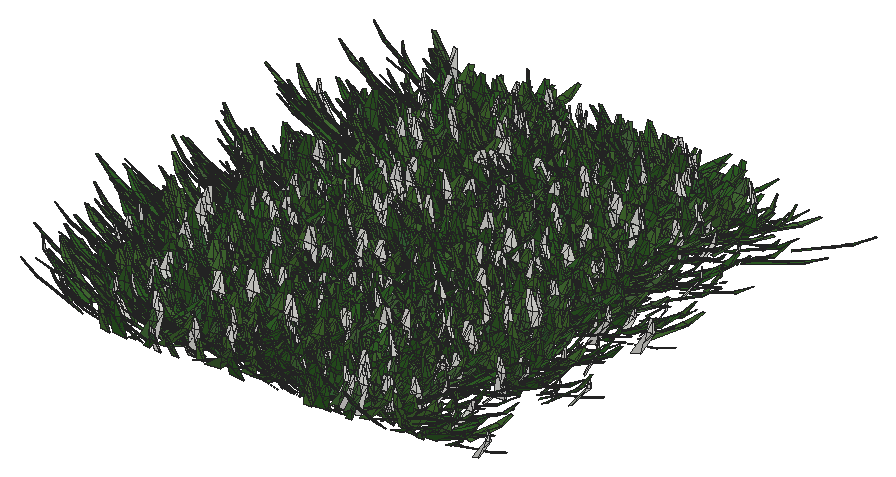
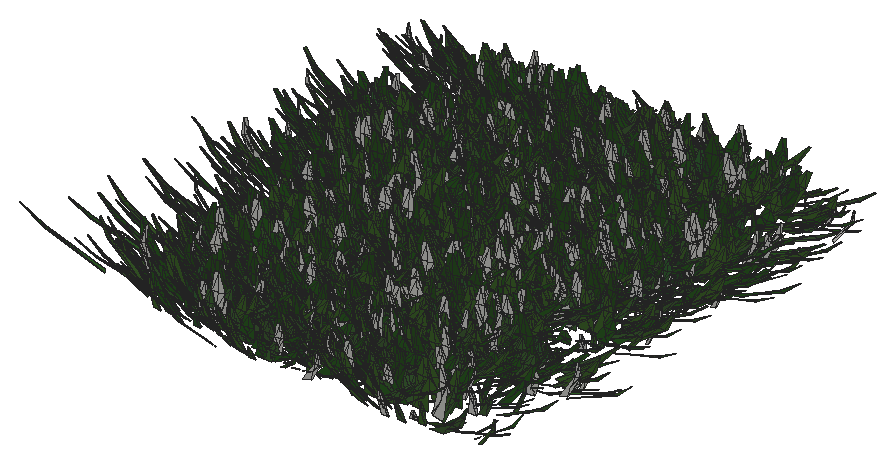
# SketchUp Ruby script. Lengths in inches.
U = 1.inch
M = Sketchup.active_model
def pt(a) = Geom::Point3d.new(a.map { |v| v * U })
def face(e, loops, mat)
  f = e.add_face(loops[0].map { |a| pt(a) })
  loops[1..].each { |l| e.add_face(l.map { |a| pt(a) }).erase! }
  f.material = f.back_material = mat if mat
  f
end
# faces: each face lists its corners as indices into pts; further lists are holes
def faces(e, pts, list, mat = nil) = list.each { |f| face(e, (f[0].is_a?(Array) ? f : [f]).map { |l| l.map { |i| pts[i] } }, mat) }
# xy, xz, yz: faces in a plane at the given z, y or x. An outline is a flat list of corners, or four numbers for a rectangle; further outlines are holes
def ring(l) = l.size == 4 ? [[l[0], l[1]], [l[2], l[1]], [l[2], l[3]], [l[0], l[3]]] : l.each_slice(2).to_a
def flat(e, list, mat, &to3) = list.each { |f| face(e, (f[0].is_a?(Array) ? f : [f]).map { |l| ring(l).map { |u, v| to3.(u, v) } }, mat) }
def xy(e, z, list, mat = nil) = flat(e, list, mat) { |x, y| [x, y, z] }
def xz(e, y, list, mat = nil) = flat(e, list, mat) { |x, z| [x, y, z] }
def yz(e, x, list, mat = nil) = flat(e, list, mat) { |y, z| [x, y, z] }
def lines(e, pts, list) = list.each { |a, b| e.add_line(pt(pts[a]), pt(pts[b])) }
# prism: a flat outline (further loops are holes) pulled along v
def prism(e, loops, v, mat = nil)
  f = face(e, loops, mat); d = Geom::Vector3d.new(v.map { |x| x * U })
  f.pushpull(f.normal.samedirection?(d) ? d.length : -d.length)
end
def box(e, o, s, mat = nil) = prism(e, [[o, [o[0] + s[0], o[1], o[2]], [o[0] + s[0], o[1] + s[1], o[2]], [o[0], o[1] + s[1], o[2]]]], [0, 0, s[2]], mat)
def at(x, y, z, deg = 0) = Geom::Transformation.translation(pt([x, y, z])) * Geom::Transformation.rotation(ORIGIN, Z_AXIS, deg.degrees)
def axes(o, x, y, z) = Geom::Transformation.new([*x, 0, *y, 0, *z, 0, *pt(o).to_a, 1])
def part(name) = M.definitions.add(name)
# library, detail: a bought-in or finely detailed component or shape, given as its bounding box
def library(name, o, s) = part(name).tap { |d| box(d.entities, o, s) }
def detail(e, o, s) = box(e.add_group.entities, o, s)
def put(e, d, t, mat = nil) = e.add_instance(d, t).tap { |i| i.material = mat if mat }
def group(e, t, mat = nil) = e.add_group.tap { |g| g.transformation = t; g.material = mat if mat }.entities
root = M.entities
M.materials.add("Material10").color = [48, 100, 38]
M.materials.add("Material3").color = [68, 110, 58]
M.materials.add("Material4").color = [48, 90, 38]
M.materials.add("Material5").color = [68, 110, 48]
M.materials.add("Material6").color = [48, 90, 48]
M.materials.add("Material7").color = [58, 110, 58]
M.materials.add("Material8").color = [58, 90, 38]
M.materials.add("Material9").color = [68, 100, 58]
c1 = part("grass00")
p = [[-0.6875,0.15,0],[-0.56,0.08,5.52],[-0.04,0.03,2.76],[0.48,-0.02,0],[0.35,-0.02,5.52],[-0.1,-0.14,5.52],
  [-0.12,0.65,8.37],[-0.42,0.65,8.37]]
faces(c1.entities,p,[[0,1,2,3],[3,2,4],[1,5,2],[5,4,2],[1,6,5],[4,5,6],[7,6,1]])
c2 = part("Group16\#1")
put(c2.entities,c1,axes([1.44,-0.61,-0.01],[0.05352,0.12609,0],[-0.10704,0.04543,0.07239],[0.06664,-0.02828,0.11628]),"Material6")
put(c2.entities,c1,axes([0.76,-0.15,-0.01],[0.04676,0.24062,0],[-0.23162,0.04501,0.06642],[0.0652,-0.01267,0.23595]),"Material3")
put(c2.entities,c1,axes([0.79,0.01,-0.01],[-0.00606,0.34651,0],[-0.34381,-0.00602,0.0432],[0.04319,0.00076,0.34386]))
put(c2.entities,c1,axes([1,0.23,-0.01],[-0.07192,0.31144,0],[-0.28722,-0.06632,0.1236],[0.12043,0.02781,0.29478]),"Material5")
put(c2.entities,c1,axes([1.66,0.77,-0.01],[-0.13828,0.29651,0],[-0.21551,-0.1005,0.22471],[0.20365,0.09498,0.23779]),"Material10")
put(c2.entities,c1,axes([0.6875,0.52,-0.01],[-0.18126,0.24051,0],[-0.22746,-0.17142,0.09788],[0.07817,0.05891,0.28481]),"Material5")
put(c2.entities,c1,axes([0.68,0.78,-0.01],[-0.215,0.18688,0],[-0.12385,-0.14248,0.21334],[0.13995,0.16101,0.18878]),"Material3")
put(c2.entities,c1,axes([0.56,1,-0.01],[-0.13756,0.07624,0],[-0.06159,-0.11112,0.0927],[0.04494,0.08108,0.12705]),"Material5")
put(c2.entities,c1,axes([0.2,0.64,-0.01],[-0.23729,0.07254,0],[-0.05711,-0.18681,0.153],[0.04473,0.14632,0.19535]),"Material10")
put(c2.entities,c1,axes([0.0625,0.72,-0.01],[-0.28874,0.02525,0],[-0.02179,-0.24916,0.14647],[0.01276,0.14591,0.25012]),"Material3")
put(c2.entities,c1,axes([-0.08,0.62,-0.01],[-0.34089,-0.04187,0],[0.03255,-0.26504,0.216],[-0.02633,0.21439,0.26703]),"Material10")
put(c2.entities,c1,axes([-0.34,0.98,-0.01],[-0.14314,-0.0493,0],[0.04397,-0.12769,0.06843],[-0.02228,0.0647,0.13505]),"Material10")
put(c2.entities,c1,axes([-0.87,1.45,-0.01],[-0.23488,-0.14114,0],[0.13761,-0.22901,0.06087],[-0.03135,0.05217,0.26717]))
put(c2.entities,c1,axes([-0.72,0.77,-0.01],[-0.14208,-0.13251,0],[0.07209,-0.0773,0.16301],[-0.11118,0.11922,0.1057]),"Material10")
put(c2.entities,c1,axes([-0.62,0.43,-0.01],[-0.14845,-0.21203,0],[0.18654,-0.13061,0.12304],[-0.10079,0.07057,0.22772]),"Material3")
put(c2.entities,c1,axes([-0.68,0.29,-0.01],[-0.13639,-0.32136,0],[0.31723,-0.13464,0.05579],[-0.05136,0.0218,0.34462]),"Material4")
put(c2.entities,c1,axes([-0.64,0.125,-0.01],[-0.0458,-0.23569,0],[0.22124,-0.043,0.08276],[-0.08124,0.01579,0.22538]),"Material7")
put(c2.entities,c1,axes([-1.6,-0.03,-0.01],[0.00576,-0.32897,0],[0.27526,0.00482,0.18018],[-0.18015,-0.00315,0.2753]),"Material5")
put(c2.entities,c1,axes([-1.36,-0.31,-0.01],[0.05718,-0.24765,0],[0.18172,0.04196,0.17267],[-0.16825,-0.03885,0.1865]),"Material10")
put(c2.entities,c1,axes([-1.54,-0.72,-0.01],[0.06537,-0.14017,0],[0.13555,0.06321,0.03939],[-0.0357,-0.01665,0.14956]))
put(c2.entities,c1,axes([-1.19,-0.9,-0.01],[0.09597,-0.12735,0],[0.11214,0.08451,0.07557],[-0.06035,-0.04548,0.14042]),"Material9")
put(c2.entities,c1,axes([-0.47,-0.54,-0.01],[0.11588,-0.10072,0],[0.0618,0.0711,0.12124],[-0.07953,-0.0915,0.0942]))
put(c2.entities,c1,axes([-0.47,-0.84,-0.01],[0.11927,-0.0661,0],[0.06603,0.11913,0.00646],[-0.00313,-0.00565,0.13621]),"Material5")
put(c2.entities,c1,axes([-0.38,-1.24,-0.01],[0.28037,-0.08571,0],[0.0618,0.20215,0.20315],[-0.05939,-0.19428,0.21139]),"Material9")
put(c2.entities,c1,axes([-0.06,-0.66,-0.01],[0.22719,-0.01987,0],[0.01247,0.14255,0.17758],[-0.01547,-0.17691,0.1431]),"Material8")
put(c2.entities,c1,axes([0.11,-0.89,-0.01],[0.14882,0.01828,0],[-0.01058,0.08611,0.12229],[0.01491,-0.12138,0.08676]),"Material6")
put(c2.entities,c1,axes([0.25,-0.72,-0.01],[0.20481,0.07053,0],[-0.06206,0.18022,0.10291],[0.03351,-0.0973,0.1906]),"Material6")
put(c2.entities,c1,axes([0.85,-1.42,-0.01],[0.16481,0.09904,0],[-0.09472,0.15762,0.05616],[0.02893,-0.04814,0.18389]),"Material5")
put(c2.entities,c1,axes([1.01,-1.09,-0.01],[0.21858,0.20385,0],[-0.17495,0.1876,0.15339],[0.10462,-0.11218,0.25652]),"Material10")
put(c2.entities,c1,axes([1.01,-0.71,-0.01],[0.08733,0.12473,0],[-0.06445,0.04512,0.13037],[0.1068,-0.07477,0.07867]),"Material6")
c3 = part("Group15\#1")
put(c3.entities,c2,at(0,0,0))
c4 = part("3darcstudiotree_grass00\#1")
put(c4.entities,c3,at(0,0,0))
put(root,c4,axes([859.57,954.71,0],[0.26147,-1.07741,0],[4.77538,0.07243,-0.04584],[0.20115,0.00305,1.3146]))
put(root,c4,axes([859.86,942.64,0],[-0.00527,-1.07979,0],[5.08619,-0.00155,-0.02113],[0.09419,-0.00003,1.41674]))
put(root,c4,axes([858.4,937.72,0],[3.80252,-0.21307,0],[0.8211,0.91584,-0.01015],[0.01463,0.01631,1.54623]))
put(root,c4,axes([858.36,939.11,0],[-1.38358,0.95904,0],[-3.87916,-0.34977,-0.00809],[-0.05318,-0.0048,1.80065]))
put(root,c4,axes([860.09,972.71,0],[-2.64683,-0.75591,0],[3.71627,-0.81329,-0.03006],[0.12697,-0.02779,1.73276]))
put(root,c4,axes([859.0625,943.74,0],[3.22127,-0.6295,0],[2.94777,0.94277,-0.00613],[0.02206,0.00705,1.74641]))
put(root,c4,axes([858.26,952.51,0],[0.12956,0.95583,0],[-3.83664,0.0325,-0.00216],[-0.01582,0.00013,1.758]))
put(root,c4,axes([859.75,968.45,0],[0.29566,-0.96452,0],[4.47879,0.08581,-0.05496],[0.37486,0.00718,1.9204]))
put(root,c4,axes([860.07,946.03,0],[-0.81018,-1.00031,0],[4.10104,-0.2076,-0.04711],[0.26622,-0.01348,1.50792]))
put(root,c4,axes([859.15,960.93,0],[3.64126,-0.56822,0],[2.32111,0.92964,-0.03499],[0.12777,0.05117,1.88939]))
put(root,c4,axes([859.51,949.74,0],[2.71786,-0.72349,0],[3.02088,0.70927,-0.02466],[0.11069,0.02599,1.59511]))
put(root,c4,axes([859.33,940.95,0],[-3.07818,0.70756,0],[-3.19663,-0.86917,-0.0061],[-0.02564,-0.00697,1.83281]))
put(root,c4,axes([859.26,936.04,0],[-1.05333,1.02923,0],[-4.06109,-0.25976,-0.04208],[-0.23965,-0.01533,1.54007]))
put(root,c4,axes([860.87,948.46,0],[-0.35317,-0.93176,0],[5.0183,-0.11888,-0.03587],[0.18182,-0.00431,1.60406]))
put(root,c4,axes([859.13,929.75,0],[0.93736,0.93245,0],[-4.81106,0.30227,-0.04255],[-0.20854,0.0131,1.5668]))
put(root,c4,axes([859.34,963.21,0],[4.77949,0.09804,0],[-0.30213,0.92053,-0.01884],[-0.00915,0.02789,1.37151]))
put(root,c4,axes([859.22,962.51,0],[3.18507,0.78996,0],[-2.86494,0.72195,-0.02475],[-0.11175,0.02816,1.62992]))
put(root,c4,axes([859.48,935.36,0],[4.28562,0.46278,0],[-1.51887,0.87911,-0.02193],[-0.0534,0.03091,1.47013]))
put(root,c4,axes([860.44,926.77,0],[3.286,-0.8357,0],[2.84385,0.69888,-0.02297],[0.11018,0.02708,1.67632]))
put(root,c4,axes([860.38,933.74,0],[4.17584,-0.76775,0],[2.82757,0.96121,-0.02397],[0.06306,0.02144,1.32443]))
put(root,c4,axes([860.375,951.46,0],[4.18652,-0.74489,0],[2.19035,0.7694,-0.02041],[0.09799,0.03442,1.95445]))
put(root,c4,axes([860.22,947.05,0],[4.0539,0.02185,0],[-0.08547,0.99116,-0.0399],[-0.00654,0.07588,1.8861]))
put(root,c4,axes([863.26,961.08,0],[-1.7872,-0.89941,0],[4.01851,-0.49907,-0.01655],[0.09453,-0.01174,1.78815]))
put(root,c4,axes([864.54,964.71,0],[-3.91628,-0.80857,0],[3.0662,-0.92819,-0.02974],[0.08498,-0.02572,1.35064]))
put(root,c4,axes([864.26,945.11,0],[-0.87255,-1.13865,0],[3.68469,-0.17647,-0.01579],[0.09603,-0.0046,1.45182]))
put(root,c4,axes([863.32,930.36,0],[-2.48301,0.65721,0],[-3.57154,-0.84335,-0.01576],[-0.06998,-0.01652,1.87507]))
put(root,c4,axes([864.8125,942.05,0],[-4.92325,-0.27664,0],[0.91141,-1.01375,-0.03373],[0.03797,-0.04223,1.33323]))
put(root,c4,axes([864.73,943.58,0],[-5.12565,0.19811,0],[-0.59233,-0.95782,-0.03554],[-0.04116,-0.06655,1.83631]))
put(root,c4,axes([863.33,948.08,0],[-0.11297,1.08035,0],[-4.48718,-0.02933,-0.03889],[-0.20921,-0.00137,1.50954]))
put(root,c4,axes([864.23,946.62,0],[-3.61171,0.88239,0],[-2.76709,-0.70787,-0.01484],[-0.07769,-0.01988,1.85373]))
put(root,c4,axes([864.37,951.24,0],[2.72646,-0.79563,0],[3.21066,0.68764,-0.00664],[0.02825,0.00605,1.48048]))
put(root,c4,axes([863.375,962.62,0],[0.71242,1.197,0],[-3.75762,0.13978,-0.01524],[-0.1206,0.00449,1.90022]))
put(root,c4,axes([864.93,928.29,0],[-3.78089,0.19176,0],[-0.79047,-0.97412,-0.01756],[-0.02482,-0.03059,1.76676]))
put(root,c4,axes([864.59,958.56,0],[-3.36041,0.90799,0],[-3.17072,-0.73341,-0.0352],[-0.15551,-0.03597,1.62511]))
put(root,c4,axes([864.93,931.68,0],[0.85917,-1.09149,0],[4.23857,0.20853,-0.05061],[0.35882,0.01765,1.95081]))
put(root,c4,axes([864.05,967.85,0],[2.92569,0.54408,0],[-2.20569,0.74129,-0.0148],[-0.07382,0.02481,1.93047]))
put(root,c4,axes([865.95,954.37,0],[-1.3197,-0.88454,0],[4.35554,-0.40614,-0.0406],[0.24185,-0.02255,1.84742]))
put(root,c4,axes([865.02,939.75,0],[-0.61826,0.98554,0],[-3.83572,-0.15039,-0.01794],[-0.11657,-0.00457,1.59592]))
put(root,c4,axes([865.07,966.49,0],[4.34755,0.01968,0],[-0.0883,1.21931,-0.04973],[-0.00561,0.07747,1.89995]))
put(root,c4,axes([864.99,953.61,0],[2.15023,1.14351,0],[-3.90551,0.45899,-0.03464],[-0.20705,0.02433,1.78143]))
put(root,c4,axes([866.24,933.27,0],[1.77249,-0.83828,0],[4.36469,0.5768,-0.05061],[0.28357,0.03747,1.95538]))
put(root,c4,axes([865.43,971.69,0],[1.34979,0.94972,0],[-3.68739,0.32754,-0.0026],[-0.01469,0.00131,1.46428]))
put(root,c4,axes([867.47,934.92,0],[-2.47748,-1.01613,0],[3.676,-0.56016,-0.05337],[0.25605,-0.03902,1.5119]))
put(root,c4,axes([867.63,958.04,0],[-2.66833,-0.96931,0],[3.87821,-0.66725,-0.05298],[0.21893,-0.03767,1.4759]))
put(root,c4,axes([866.98,949.71,0],[2.30666,-1.0875,0],[4.46305,0.59165,-0.05067],[0.21491,0.02849,1.51576]))
put(root,c4,axes([866.875,936.16,0],[2.28163,-1.10876,0],[3.45513,0.44438,-0.03693],[0.24001,0.03087,1.77491]))
put(root,c4,axes([865.83,940.95,0],[0.86518,1.01256,0],[-4.67116,0.24945,-0.00171],[-0.00978,0.00052,1.74655]))
put(root,c4,axes([867.71,956.47,0],[1.85636,-0.87548,0],[4.2252,0.55994,-0.01977],[0.10435,0.01383,1.78562]))
put(root,c4,axes([866.46,937.46,0],[3.65118,0.22835,0],[-1.21465,1.21387,-0.00744],[-0.00809,0.00808,1.4009]))
put(root,c4,axes([866.96,969.63,0],[3.69854,-0.02221,0],[0.11187,1.16446,-0.04057],[0.00448,0.0466,1.33829]))
put(root,c4,axes([867.1,927.01,0],[3.07982,0.93534,0],[-3.08003,0.63386,-0.01155],[-0.0607,0.01249,1.69697]))
put(root,c4,axes([867.68,963.56,0],[1.29993,0.864,0],[-3.89937,0.36667,-0.04913],[-0.3212,0.0302,1.81865]))
put(root,c4,axes([869.47,968.03,0],[-4.57324,0.06463,0],[-0.23944,-1.05899,-0.00256],[-0.00093,-0.0041,1.70382]))
put(root,c4,axes([870.29,963.2,0],[-0.89657,-1.00818,0],[4.16611,-0.23156,-0.01455],[0.07266,-0.00404,1.36448]))
put(root,c4,axes([870.52,940.95,0],[-4.48956,-0.10603,0],[0.4036,-1.06805,-0.03137],[0.01455,-0.03851,1.3228]))
put(root,c4,axes([869.92,953.04,0],[-3.51738,0.88979,0],[-2.84475,-0.70284,-0.03007],[-0.16867,-0.04167,1.97134]))
put(root,c4,axes([871.01,946.53,0],[-1.66366,-1.09388,0],[4.81129,-0.45734,-0.02869],[0.11735,-0.01115,1.40786]))
put(root,c4,axes([870.93,966.48,0],[-3.48279,-0.87064,0],[3.22991,-0.80753,-0.05204],[0.22842,-0.05711,1.77215]))
put(root,c4,axes([871.16,929.125,0],[-3.93857,-0.30978,0],[1.37085,-1.08932,-0.00258],[0.00367,-0.00291,1.35273]))
put(root,c4,axes([869.875,957.91,0],[3.6556,-0.00646,0],[0.03301,1.16694,-0.0442],[0.00143,0.05063,1.33678]))
put(root,c4,axes([871.19,969.25,0],[-0.76209,-0.8955,0],[4.21088,-0.22397,-0.04713],[0.27128,-0.01443,1.58351]))
put(root,c4,axes([870.92,931.82,0],[2.17212,-0.7546,0],[4.09706,0.73708,-0.05142],[0.26111,0.04697,1.97373]))
put(root,c4,axes([871.42,936.23,0],[-4.62143,0.243,0],[-0.94962,-1.12878,-0.01674],[-0.02169,-0.02578,1.81501]))
put(root,c4,axes([870.73,949.55,0],[-1.86129,1.04113,0],[-3.56127,-0.39792,-0.0353],[-0.23679,-0.02646,1.79152]))
put(root,c4,axes([870.09,959.12,0],[-0.25494,0.97633,0],[-4.14,-0.06757,-0.01044],[-0.06049,-0.00099,1.50484]))
put(root,c4,axes([870.69,948.8125,0],[-1.81241,0.85441,0],[-3.27922,-0.43475,-0.02105],[-0.15086,-0.02,1.88169]))
put(root,c4,axes([871.83,927.52,0],[-1.30769,-0.93335,0],[3.48924,-0.30554,-0.02961],[0.16247,-0.01423,1.34337]))
put(root,c4,axes([869.96,939.56,0],[3.58871,0.50463,0],[-2.17344,0.96603,-0.00275],[-0.00669,0.00297,1.37565]))
put(root,c4,axes([872.09,942.04,0],[-3.15251,-0.61197,0],[3.07523,-0.99011,-0.06125],[0.16311,-0.05251,1.36064]))
put(root,c4,axes([871.6,945.52,0],[0.12937,-1.28679,0],[4.29461,0.02699,-0.05528],[0.32895,0.00207,1.59813]))
put(root,c4,axes([870.71,960.48,0],[-1.95389,0.95896,0],[-4.54088,-0.57825,-0.01882],[-0.07855,-0.01,1.49212]))
put(root,c4,axes([872.68,964.93,0],[0.30161,-1.10509,0],[5.10821,0.08714,-0.02398],[0.09779,0.00167,1.30813]))
put(root,c4,axes([872.21,970.92,0],[-4.48167,0.42231,0],[-1.44453,-0.9581,-0.00238],[-0.00433,-0.00287,1.31717]))
put(root,c4,axes([871.39,929.83,0],[3.80777,-0.2002,0],[0.96857,1.15138,-0.04208],[0.03932,0.04675,1.3356]))
put(root,c4,axes([873.09,951.9,0],[-1.21535,-0.91451,0],[3.60544,-0.29947,-0.00285],[0.02203,-0.00183,1.93438]))
put(root,c4,axes([873.05,944.04,0],[-2.37468,-0.98502,0],[3.18628,-0.48009,-0.03107],[0.19051,-0.0287,1.66455]))
put(root,c4,axes([873.31,955.07,0],[-4.21878,-0.13998,0],[0.64353,-1.21222,-0.01228],[0.00866,-0.0163,1.63767]))
put(root,c4,axes([873.41,934.83,0],[0.48505,-1.08337,0],[4.27123,0.11952,-0.04376],[0.24596,0.00688,1.51939]))
put(root,c4,axes([872.86,962.61,0],[-2.73895,0.66336,0],[-3.26902,-0.84359,-0.02879],[-0.12001,-0.03097,1.7592]))
put(root,c4,axes([872.98,933.52,0],[-2.4816,0.92551,0],[-3.41349,-0.57204,-0.02214],[-0.11703,-0.01961,1.63462]))
put(root,c4,axes([873.36,955.89,0],[-1.82662,0.77889,0],[-3.91562,-0.57392,-0.01566],[-0.07709,-0.0113,1.61828]))
put(root,c4,axes([873.47,937.8,0],[4.05704,-0.60104,0],[1.84911,0.7801,-0.02001],[0.07729,0.03261,1.71774]))
put(root,c4,axes([875.45,968.55,0],[-3.56139,-0.59682,0],[2.57727,-0.96121,-0.05337],[0.16285,-0.06074,1.58535]))
put(root,c4,axes([876.62,970.2,0],[-3.83504,-0.49614,0],[2.03803,-0.98459,-0.02021],[0.06424,-0.03103,1.91641]))
put(root,c4,axes([876.92,965.32,0],[0.25783,-1.11098,0],[4.27668,0.06203,-0.02273],[0.12742,0.00185,1.50351]))
put(root,c4,axes([877.1875,928.43,0],[-4.85,-0.22958,0],[0.83383,-1.10092,-0.02653],[0.02986,-0.03943,1.69452]))
put(root,c4,axes([876.18,963.94,0],[4.62804,-0.23272,0],[0.89278,1.10968,-0.02659],[0.02814,0.03498,1.51897]))
put(root,c4,axes([878.21,955.125,0],[-4.56641,-0.61307,0],[2.03224,-0.94607,-0.02099],[0.05514,-0.02567,1.49075]))
put(root,c4,axes([876.19,972.44,0],[3.22508,0.4199,0],[-2.23997,1.07528,-0.0178],[-0.0355,0.01704,1.30843]))
put(root,c4,axes([877.37,942.74,0],[2.46228,-0.71132,0],[3.57586,0.77364,-0.03846],[0.1554,0.03362,1.57923]))
put(root,c4,axes([878.08,929.89,0],[-3.78747,-0.21466,0],[0.95822,-1.0567,-0.03754],[0.05955,-0.06567,1.94323]))
put(root,c4,axes([878.19,955.75,0],[-2.12409,-0.80452,0],[3.07899,-0.50807,-0.03406],[0.21345,-0.03522,1.73123]))
put(root,c4,axes([878.58,941.08,0],[-2.37888,-1.01371,0],[3.74365,-0.54908,-0.03431],[0.16796,-0.02463,1.53951]))
put(root,c4,axes([877.85,949.9,0],[2.88746,-1.01127,0],[4.01064,0.71572,-0.04124],[0.17013,0.03036,1.56101]))
put(root,c4,axes([878.2,959.05,0],[0.65857,-1.17921,0],[3.67761,0.12837,-0.0384],[0.25113,0.00877,1.53253]))
put(root,c4,axes([877.3,948.89,0],[3.72974,0.07459,0],[-0.38183,1.19325,-0.00093],[-0.00033,0.00104,1.35201]))
put(root,c4,axes([876.99,939.55,0],[4.3834,0.50633,0],[-1.68665,0.91261,-0.00765],[-0.01741,0.00942,1.36419]))
put(root,c4,axes([878.99,952.74,0],[0.55792,-1.05016,0],[4.92434,0.16351,-0.03191],[0.17517,0.00582,1.71939]))
put(root,c4,axes([879.27,936.47,0],[-4.56826,-0.36259,0],[1.35513,-1.06708,-0.0262],[0.03858,-0.03038,1.36239]))
put(root,c4,axes([877.05,966.56,0],[4.02014,0.68076,0],[-2.86441,1.05721,-0.02464],[-0.08583,0.03168,1.98292]))
put(root,c4,axes([879.26,944.92,0],[-3.83129,-0.35772,0],[1.74028,-1.16494,-0.03885],[0.07795,-0.05218,1.78292]))
put(root,c4,axes([877.37,951.01,0],[-0.31476,0.91274,0],[-4.84329,-0.10439,-0.00545],[-0.03468,-0.00075,1.93955]))
put(root,c4,axes([877.82,933.04,0],[4.30418,0.00494,0],[-0.017,0.92497,-0.03904],[-0.00144,0.07818,1.85207]))
put(root,c4,axes([878.38,960.44,0],[-1.66993,0.87259,0],[-3.97117,-0.47499,-0.02774],[-0.12868,-0.01539,1.41462]))
put(root,c4,axes([877.56,961.79,0],[3.65221,0.81587,0],[-2.94048,0.82269,-0.00121],[-0.00437,0.00122,1.48985]))
put(root,c4,axes([879.72,946.69,0],[-4.23214,-0.05547,0],[0.1952,-0.93083,-0.00586],[0.00226,-0.01076,1.71352]))
put(root,c4,axes([878.16,943.97,0],[0.83957,1.19196,0],[-3.66821,0.16148,-0.02162],[-0.1209,0.00532,1.32159]))
put(root,c4,axes([878.55,971.1875,0],[3.80473,0.13574,0],[-0.67195,1.17716,-0.03434],[-0.02787,0.04883,1.70799]))
put(root,c4,axes([879,927.36,0],[3.39209,-0.30668,0],[1.53109,1.05845,-0.04794],[0.07887,0.05453,1.36124]))
put(root,c4,axes([878.27,957.67,0],[4.29167,0.73108,0],[-2.5905,0.95044,-0.06012],[-0.15898,0.05833,1.3502]))
put(root,c4,axes([879.42,931.46,0],[4.6588,-0.38386,0],[1.34446,1.01982,-0.0158],[0.03633,0.02756,1.97161]))
put(root,c4,axes([879.04,934.31,0],[0.81792,0.98803,0],[-4.75058,0.24579,-0.00233],[-0.01332,0.00069,1.77271]))
put(root,c4,axes([879.54,938.34,0],[3.79999,0.06244,0],[-0.29859,1.1358,-0.01423],[-0.00601,0.02286,1.83161]))
put(root,c4,axes([882.01,936.74,0],[-4.93822,-0.11046,0],[0.42261,-1.18087,-0.03473],[0.01792,-0.05006,1.7157]))
put(root,c4,axes([881.41,927.35,0],[2.61594,-0.62324,0],[2.61447,0.68586,-0.03437],[0.16704,0.04382,1.66865]))
put(root,c4,axes([882.18,930.21,0],[0.42125,-1.19943,0],[4.10961,0.09021,-0.02351],[0.14993,0.00329,1.65028]))
put(root,c4,axes([882.4,962.43,0],[0.15957,-0.94034,0],[4.98466,0.05287,-0.04061],[0.22246,0.00236,1.70991]))
put(root,c4,axes([882.75,946.57,0],[-1.41294,-1.10212,0],[4.32228,-0.34633,-0.03893],[0.21471,-0.0172,1.64312]))
put(root,c4,axes([883.04,948.45,0],[-3.69312,-0.8813,0],[3.34955,-0.87728,-0.04863],[0.21671,-0.05676,1.95701]))
put(root,c4,axes([882.82,934.35,0],[-0.87663,-1.01395,0],[4.66847,-0.25226,-0.06129],[0.26842,-0.0145,1.3376]))
put(root,c4,axes([881.99,966.87,0],[3.5325,-0.69831,0],[2.94663,0.93162,-0.01988],[0.08154,0.02578,1.96304]))
put(root,c4,axes([882.75,954.72,0],[0.77857,-0.99525,0],[5.0673,0.24776,-0.06032],[0.25875,0.01265,1.41053]))
put(root,c4,axes([882.79,950.3,0],[-3.85062,-0.01072,0],[0.0412,-0.92486,-0.02017],[0.00173,-0.03873,1.77597]))
put(root,c4,axes([883.4,937.73,0],[-2.58333,-1.04048,0],[3.69668,-0.57364,-0.02087],[0.10332,-0.01603,1.58468]))
put(root,c4,axes([883.14,968.51,0],[-3.948,-0.1076,0],[0.50589,-1.16017,-0.01401],[0.009,-0.02065,1.72979]))
put(root,c4,axes([883.5625,964.22,0],[-5.08538,0.01363,0],[-0.0515,-1.20054,-0.01941],[-0.00134,-0.03118,1.92834]))
put(root,c4,axes([883.67,931.27,0],[-4.60962,0.0959,0],[-0.32649,-0.98088,-0.01346],[-0.00781,-0.02346,1.72106]))
put(root,c4,axes([882.35,960.25,0],[4.17924,-0.09662,0],[0.4087,1.10487,-0.00914],[0.00578,0.01563,1.90465]))
put(root,c4,axes([882.44,941.24,0],[2.55931,1.04661,0],[-3.2663,0.4992,-0.02868],[-0.15491,0.02367,1.51486]))
put(root,c4,axes([884.4375,957.5625,0],[-0.89831,-1.0989,0],[4.77812,-0.24412,-0.03636],[0.19134,-0.00978,1.63697]))
put(root,c4,axes([883.5,970.71,0],[-2.18401,1.00403,0],[-3.62225,-0.49246,-0.03157],[-0.1939,-0.02636,1.80167]))
put(root,c4,axes([883.0625,933.27,0],[3.60668,0.39506,0],[-2.04442,1.16653,-0.0492],[-0.09575,0.05464,1.54416]))
put(root,c4,axes([883.54,965.35,0],[4.80917,-0.20992,0],[0.88931,1.27332,-0.04063],[0.03159,0.04524,1.46079]))
put(root,c4,axes([884.94,928.72,0],[1.09083,-0.85917,0],[4.87884,0.38714,-0.04397],[0.18771,0.0149,1.43296]))
put(root,c4,axes([885.36,939.82,0],[0.74314,-1.27426,0],[5.01119,0.18265,-0.00277],[0.01296,0.00047,1.49508]))
put(root,c4,axes([883.73,955.52,0],[4.05871,-0.05513,0],[0.21483,0.98855,-0.02262],[0.008,0.03681,1.6131]))
put(root,c4,axes([883.87,942.45,0],[2.41461,0.82437,0],[-3.20063,0.58592,-0.01948],[-0.10927,0.02,1.72408]))
put(root,c4,axes([885.58,951.67,0],[-4.13654,0.57707,0],[-2.0044,-0.898,-0.03544],[-0.10461,-0.04686,1.55733]))
put(root,c4,axes([885.68,945,0],[2.18961,-0.72887,0],[3.37602,0.63387,-0.00267],[0.01513,0.00284,1.87177]))
put(root,c4,axes([885.87,953.38,0],[-4.20241,0.23168,0],[-1.01309,-1.14851,-0.02531],[-0.03283,-0.03722,1.77094]))
put(root,c4,axes([884.48,944.09,0],[3.66493,0.77131,0],[-3.09992,0.92059,-0.01247],[-0.04973,0.01477,1.86292]))
put(root,c4,axes([885.79,969.32,0],[4.71809,-0.16737,0],[0.67524,1.18967,-0.05794],[0.04945,0.08711,1.82474]))
put(root,c4,axes([887.68,949.48,0],[-3.89812,-0.79774,0],[2.64275,-0.80711,-0.04086],[0.17451,-0.0533,1.75811]))
put(root,c4,axes([885.65,959.5,0],[0.07283,1.03714,0],[-5.06058,0.02221,-0.00579],[-0.03358,0.00015,1.83497]))
put(root,c4,axes([888,942.77,0],[-0.48105,-1.08782,0],[3.72041,-0.10283,-0.00454],[0.03276,-0.00091,1.6986]))
put(root,c4,axes([888.38,938.92,0],[-2.15929,-1.00318,0],[4.02891,-0.542,-0.04084],[0.19903,-0.02677,1.58232]))
put(root,c4,axes([888.6,928.36,0],[-2.83131,-0.59353,0],[3.0716,-0.91578,-0.0116],[0.03498,-0.01043,1.40225]))
put(root,c4,axes([888.18,937.99,0],[-3.84728,0.08343,0],[-0.38404,-1.1069,-0.04163],[-0.02453,-0.07069,1.89396]))
